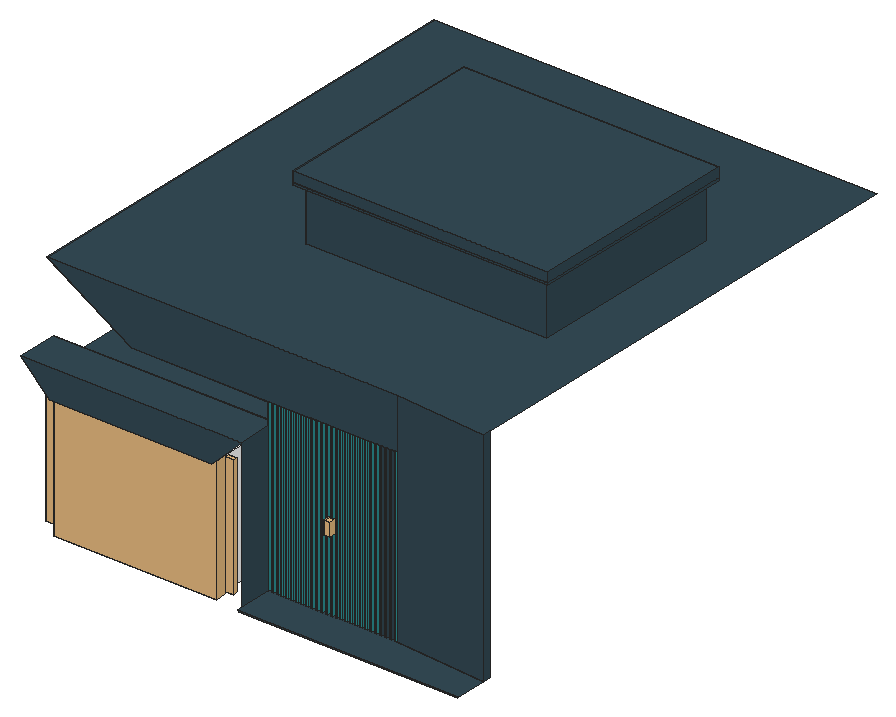
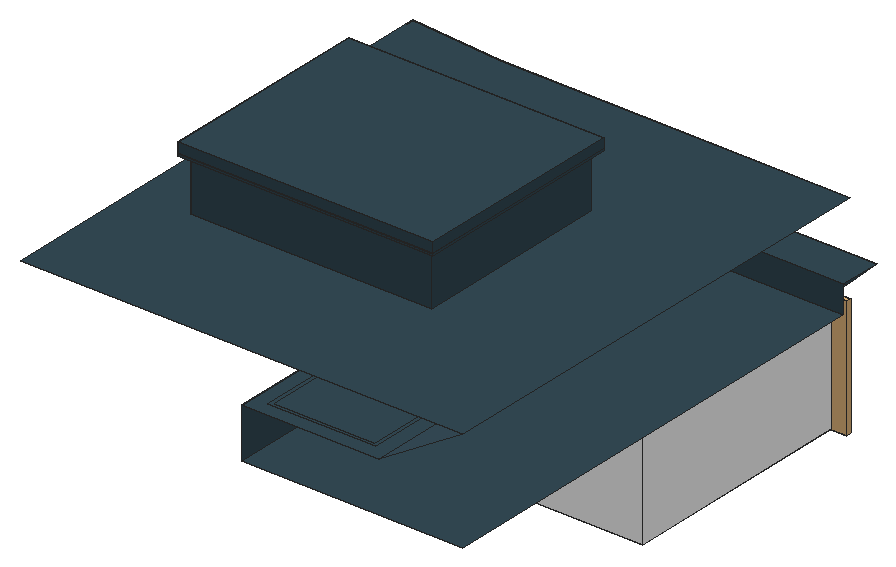
# SketchUp Ruby script. Lengths in inches.
U = 1.inch
M = Sketchup.active_model
def pt(a) = Geom::Point3d.new(a.map { |v| v * U })
def face(e, loops, mat)
  f = e.add_face(loops[0].map { |a| pt(a) })
  loops[1..].each { |l| e.add_face(l.map { |a| pt(a) }).erase! }
  f.material = f.back_material = mat if mat
  f
end
# faces: each face lists its corners as indices into pts; further lists are holes
def faces(e, pts, list, mat = nil) = list.each { |f| face(e, (f[0].is_a?(Array) ? f : [f]).map { |l| l.map { |i| pts[i] } }, mat) }
# xy, xz, yz: faces in a plane at the given z, y or x. An outline is a flat list of corners, or four numbers for a rectangle; further outlines are holes
def ring(l) = l.size == 4 ? [[l[0], l[1]], [l[2], l[1]], [l[2], l[3]], [l[0], l[3]]] : l.each_slice(2).to_a
def flat(e, list, mat, &to3) = list.each { |f| face(e, (f[0].is_a?(Array) ? f : [f]).map { |l| ring(l).map { |u, v| to3.(u, v) } }, mat) }
def xy(e, z, list, mat = nil) = flat(e, list, mat) { |x, y| [x, y, z] }
def xz(e, y, list, mat = nil) = flat(e, list, mat) { |x, z| [x, y, z] }
def yz(e, x, list, mat = nil) = flat(e, list, mat) { |y, z| [x, y, z] }
def lines(e, pts, list) = list.each { |a, b| e.add_line(pt(pts[a]), pt(pts[b])) }
# prism: a flat outline (further loops are holes) pulled along v
def prism(e, loops, v, mat = nil)
  f = face(e, loops, mat); d = Geom::Vector3d.new(v.map { |x| x * U })
  f.pushpull(f.normal.samedirection?(d) ? d.length : -d.length)
end
def box(e, o, s, mat = nil) = prism(e, [[o, [o[0] + s[0], o[1], o[2]], [o[0] + s[0], o[1] + s[1], o[2]], [o[0], o[1] + s[1], o[2]]]], [0, 0, s[2]], mat)
def at(x, y, z, deg = 0) = Geom::Transformation.translation(pt([x, y, z])) * Geom::Transformation.rotation(ORIGIN, Z_AXIS, deg.degrees)
def axes(o, x, y, z) = Geom::Transformation.new([*x, 0, *y, 0, *z, 0, *pt(o).to_a, 1])
def part(name) = M.definitions.add(name)
# library, detail: a bought-in or finely detailed component or shape, given as its bounding box
def library(name, o, s) = part(name).tap { |d| box(d.entities, o, s) }
def detail(e, o, s) = box(e.add_group.entities, o, s)
def put(e, d, t, mat = nil) = e.add_instance(d, t).tap { |i| i.material = mat if mat }
def group(e, t, mat = nil) = e.add_group.tap { |g| g.transformation = t; g.material = mat if mat }.entities
root = M.entities
M.materials.add("0466 AP 9679 Little Andaman-N").color = [89, 168, 184]
M.materials.add("0496 AP 9691 Shadow-N").color = [53, 75, 86]
M.materials.add("0502 AP 7454 DEEP TEAL").color = [46, 147, 149]
M.materials.add("[Color M00]").color = [255, 255, 255]
c1 = library("Sliding windows",[335.6875,-0.89,0.35],[144.14,8.85,122.84])
c2 = library("шторы раздвинутые\#1",[23.6875,-79.1875,2.97],[68.3125,79.67,3.21])
c3 = library("DINING SET",[25.27,8.07,0],[68.7,94.48,53.71])
c4 = library("Wall Light 02",[0,0,0],[3.15,6.76,4.53])
c5 = part("Group\#6")
xy(c5.entities,0,[[1.28,0,0.95,0.04,0.64,0.17,0.375,0.375,0.17,0.64,0.04,0.95,0,1.28,0.04,1.61,0.17,1.92,0.375,2.18,0.64,2.39,0.95,2.51,1.28,2.56,1.61,2.51,1.92,2.39,2.18,2.18,2.39,1.92,2.51,1.61,2.56,1.28,2.51,0.95,2.39,0.64,2.18,0.375,1.92,0.17,1.61,0.04]])
c6 = part("Group\#12")
detail(c6.entities,[2.45,2.45,12.38],[4,4,0.32])
put(c6.entities,c5,at(3.17,3.17,12.51),"[Color M00]")
xy(root,133,[[988.11,217.0625,1120.11,414.75]],"0496 AP 9691 Shadow-N")
xy(root,134,[[1145.11,203.25,1323.11,204.25]],"0496 AP 9691 Shadow-N")
xy(root,135,[[1144.11,203.25,1324.11,203.25,1324.11,234.25,1246.68,234.25,1246.68,236.25,1244.68,236.25,1244.68,234.25,1242.68,234.25,1242.68,236.25,1240.68,236.25,1240.68,234.25,1238.68,234.25,1238.68,236.25,1236.68,236.25,1236.68,234.25,1234.68,234.25,1234.68,236.25,1232.68,236.25,1232.68,234.25,1230.68,234.25,1230.68,236.25,1228.68,236.25,1228.68,234.25,1226.68,234.25,1226.68,236.25,1224.68,236.25,1224.68,234.25,1222.68,234.25,1222.68,236.25,1220.68,236.25,1220.68,234.25,1218.68,234.25,1218.68,236.25,1216.68,236.25,1216.68,234.25,1214.68,234.25,1214.68,236.25,1212.68,236.25,1212.68,234.25,1210.68,234.25,1210.68,236.25,1208.68,236.25,1208.68,234.25,1206.68,234.25,1206.68,236.25,1204.68,236.25,1204.68,234.25,1202.68,234.25,1202.68,236.25,1200.68,236.25,1200.68,234.25,1198.68,234.25,1198.68,236.25,1196.68,236.25,1196.68,234.25,1194.68,234.25,1194.68,236.25,1192.68,236.25,1192.68,234.25,1190.68,234.25,1190.68,236.25,1188.68,236.25,1188.68,234.25,1186.68,234.25,1186.68,236.25,1184.68,236.25,1184.68,234.25,1182.68,234.25,1182.68,236.25,1180.68,236.25,1180.68,234.25,1178.68,234.25,1178.68,236.25,1176.68,236.25,1176.68,234.25,1174.68,234.25,1174.68,236.25,1172.68,236.25,1172.68,234.25,1170.68,234.25,1170.68,236.25,1168.68,236.25,1168.68,234.25,1166.68,234.25,1166.68,236.25,1164.68,236.25,1164.68,234.25,1162.68,234.25,1162.68,236.25,1160.68,236.25,1160.68,234.25,1158.68,234.25,1158.68,236.25,1156.68,236.25,1156.68,234.25,1154.68,234.25,1154.68,236.25,1152.68,236.25,1152.68,234.25,1150.68,234.25,1150.68,236.25,1148.68,236.25,1148.68,234.25,1146.68,234.25,1146.68,236.25,1144.68,236.25,1144.68,234.25,1144.11,234.25]],"0496 AP 9691 Shadow-N")
xy(root,135.01,[[1324.11,228.25,1248.68,234.25,1324.11,234.25]],"0496 AP 9691 Shadow-N")
xy(root,231,[[988.11,207.25,1120.11,220.25]],"0496 AP 9691 Shadow-N")
xy(root,231,[[[988.11,220.25,1120.11,414.75],[1004.21,236.35,1104.01,398.65]],[1006.21,238.35,1102.01,396.65]],"[Color M00]")
xy(root,232.625,[[964.11,240.97,1144.11,627.25]],"0496 AP 9691 Shadow-N")
xy(root,255,[[964.11,207.25,1144.11,240.97]],"0496 AP 9691 Shadow-N")
xy(root,272.98,[[[1032.78,234.25,1144.11,627.25],[1044.78,246.25,1132.11,615.25]],[1144.68,234.25,1146.68,236.25],[1148.68,234.25,1150.68,236.25],[1152.68,234.25,1154.68,236.25],[1156.68,234.25,1158.68,236.25],
  [1160.68,234.25,1162.68,236.25],[1164.68,234.25,1166.68,236.25],[1168.68,234.25,1170.68,236.25],[1172.68,234.25,1174.68,236.25],[1176.68,234.25,1178.68,236.25],
  [1180.68,234.25,1182.68,236.25],[1184.68,234.25,1186.68,236.25],[1188.68,234.25,1190.68,236.25],[1192.68,234.25,1194.68,236.25],[1196.68,234.25,1198.68,236.25],
  [1200.68,234.25,1202.68,236.25],[1204.68,234.25,1206.68,236.25],[1208.68,234.25,1210.68,236.25],[1212.68,234.25,1214.68,236.25],[1216.68,234.25,1218.68,236.25],
  [1220.68,234.25,1222.68,236.25],[1224.68,234.25,1226.68,236.25],[1228.68,234.25,1230.68,236.25],[1232.68,234.25,1234.68,236.25],[1236.68,234.25,1238.68,236.25],
  [1240.68,234.25,1242.68,236.25],[1244.68,234.25,1246.68,236.25],[1046.78,248.25,1130.11,613.25]],"0496 AP 9691 Shadow-N")
xy(root,315,[[1324.11,228.25,1324.11,627.25,964.11,627.25,964.11,234.25,1248.68,234.25]],"0496 AP 9691 Shadow-N")
xz(root,207.25,[[988.11,231,1120.11,231,1144.11,255,964.11,255]],"0496 AP 9691 Shadow-N")
xz(root,234.25,[[1248.68,135,1324.11,135.01],[1248.68,135.01,1324.11,272.98],[1032.78,272.98,1248.68,272.98,1248.68,315,964.11,315]],"0496 AP 9691 Shadow-N")
xz(root,234.25,[[1144.11,135,1144.68,272.98],[1146.68,135,1148.68,272.98],[1150.68,135,1152.68,272.98],[1154.68,135,1156.68,272.98],[1158.68,135,1160.68,272.98],
  [1162.68,135,1164.68,272.98],[1166.68,135,1168.68,272.98],[1170.68,135,1172.68,272.98],[1174.68,135,1176.68,272.98],[1178.68,135,1180.68,272.98],
  [1182.68,135,1184.68,272.98],[1186.68,135,1188.68,272.98],[1190.68,135,1192.68,272.98],[1194.68,135,1196.68,272.98],[1198.68,135,1200.68,272.98],
  [1202.68,135,1204.68,272.98],[1206.68,135,1208.68,272.98],[1210.68,135,1212.68,272.98],[1214.68,135,1216.68,272.98],[1218.68,135,1220.68,272.98],
  [1222.68,135,1224.68,272.98],[1226.68,135,1228.68,272.98],[1230.68,135,1232.68,272.98],[1234.68,135,1236.68,272.98],[1238.68,135,1240.68,272.98],
  [1242.68,135,1244.68,272.98],[1246.68,135,1248.68,272.98]],"0502 AP 7454 DEEP TEAL")
xz(root,236.25,[[1144.68,135,1146.68,272.98],[1148.68,135,1150.68,272.98],[1152.68,135,1154.68,272.98],[1156.68,135,1158.68,272.98],[1160.68,135,1162.68,272.98],
  [1164.68,135,1166.68,272.98],[1168.68,135,1170.68,272.98],[1172.68,135,1174.68,272.98],[1176.68,135,1178.68,272.98],[1180.68,135,1182.68,272.98],
  [1184.68,135,1186.68,272.98],[1188.68,135,1190.68,272.98],[1192.68,135,1194.68,272.98],[1196.68,135,1198.68,272.98],[1200.68,135,1202.68,272.98],
  [1204.68,135,1206.68,272.98],[1208.68,135,1210.68,272.98],[1212.68,135,1214.68,272.98],[1216.68,135,1218.68,272.98],[1220.68,135,1222.68,272.98],
  [1224.68,135,1226.68,272.98],[1228.68,135,1230.68,272.98],[1232.68,135,1234.68,272.98],[1236.68,135,1238.68,272.98],[1240.68,135,1242.68,272.98],
  [1244.68,135,1246.68,272.98]],"0502 AP 7454 DEEP TEAL")
xz(root,240.97,[[964.11,232.625,1144.11,255]],"0496 AP 9691 Shadow-N")
xz(root,414.75,[[988.11,133,1120.11,231]],"[Color M00]")
yz(root,988.11,[[220.25,133,414.75,231]],"[Color M00]")
yz(root,1120.11,[[220.25,133,414.75,231]],"[Color M00]")
yz(root,1144.11,[[207.25,135,234.25,255],[240.97,232.625,240.97,255,234.25,255,234.25,272.98,627.25,272.98,627.25,232.625]],"0496 AP 9691 Shadow-N")
yz(root,1144.68,[[234.25,135,236.25,272.98]],"0502 AP 7454 DEEP TEAL")
yz(root,1146.68,[[234.25,135,236.25,272.98]],"0502 AP 7454 DEEP TEAL")
yz(root,1148.68,[[234.25,135,236.25,272.98]],"0502 AP 7454 DEEP TEAL")
yz(root,1150.68,[[234.25,135,236.25,272.98]],"0502 AP 7454 DEEP TEAL")
yz(root,1152.68,[[234.25,135,236.25,272.98]],"0502 AP 7454 DEEP TEAL")
yz(root,1154.68,[[234.25,135,236.25,272.98]],"0502 AP 7454 DEEP TEAL")
yz(root,1156.68,[[234.25,135,236.25,272.98]],"0502 AP 7454 DEEP TEAL")
yz(root,1158.68,[[234.25,135,236.25,272.98]],"0502 AP 7454 DEEP TEAL")
yz(root,1160.68,[[234.25,135,236.25,272.98]],"0502 AP 7454 DEEP TEAL")
yz(root,1162.68,[[234.25,135,236.25,272.98]],"0502 AP 7454 DEEP TEAL")
yz(root,1164.68,[[234.25,135,236.25,272.98]],"0502 AP 7454 DEEP TEAL")
yz(root,1166.68,[[234.25,135,236.25,272.98]],"0502 AP 7454 DEEP TEAL")
yz(root,1168.68,[[234.25,135,236.25,272.98]],"0502 AP 7454 DEEP TEAL")
yz(root,1170.68,[[234.25,135,236.25,272.98]],"0502 AP 7454 DEEP TEAL")
yz(root,1172.68,[[234.25,135,236.25,272.98]],"0502 AP 7454 DEEP TEAL")
yz(root,1174.68,[[234.25,135,236.25,272.98]],"0502 AP 7454 DEEP TEAL")
yz(root,1176.68,[[234.25,135,236.25,272.98]],"0502 AP 7454 DEEP TEAL")
yz(root,1178.68,[[234.25,135,236.25,272.98]],"0466 AP 9679 Little Andaman-N")
yz(root,1180.68,[[234.25,135,236.25,272.98]],"0502 AP 7454 DEEP TEAL")
yz(root,1182.68,[[234.25,135,236.25,272.98]],"0502 AP 7454 DEEP TEAL")
yz(root,1184.68,[[234.25,135,236.25,272.98]],"0502 AP 7454 DEEP TEAL")
yz(root,1186.68,[[234.25,135,236.25,272.98]],"0502 AP 7454 DEEP TEAL")
yz(root,1188.68,[[234.25,135,236.25,272.98]],"0502 AP 7454 DEEP TEAL")
yz(root,1190.68,[[234.25,135,236.25,272.98]],"0502 AP 7454 DEEP TEAL")
yz(root,1192.68,[[234.25,135,236.25,272.98]],"0502 AP 7454 DEEP TEAL")
yz(root,1194.68,[[234.25,135,236.25,272.98]],"0502 AP 7454 DEEP TEAL")
yz(root,1196.68,[[234.25,135,236.25,272.98]],"0502 AP 7454 DEEP TEAL")
yz(root,1198.68,[[234.25,135,236.25,272.98]],"0502 AP 7454 DEEP TEAL")
yz(root,1200.68,[[234.25,135,236.25,272.98]],"0502 AP 7454 DEEP TEAL")
yz(root,1202.68,[[234.25,135,236.25,272.98]],"0502 AP 7454 DEEP TEAL")
yz(root,1204.68,[[234.25,135,236.25,272.98]],"0502 AP 7454 DEEP TEAL")
yz(root,1206.68,[[234.25,135,236.25,272.98]],"0502 AP 7454 DEEP TEAL")
yz(root,1208.68,[[234.25,135,236.25,272.98]],"0502 AP 7454 DEEP TEAL")
yz(root,1210.68,[[234.25,135,236.25,272.98]],"0502 AP 7454 DEEP TEAL")
yz(root,1212.68,[[234.25,135,236.25,272.98]],"0502 AP 7454 DEEP TEAL")
yz(root,1214.68,[[234.25,135,236.25,272.98]],"0502 AP 7454 DEEP TEAL")
yz(root,1216.68,[[234.25,135,236.25,272.98]],"0502 AP 7454 DEEP TEAL")
yz(root,1218.68,[[234.25,135,236.25,272.98]],"0502 AP 7454 DEEP TEAL")
yz(root,1220.68,[[234.25,135,236.25,272.98]],"0502 AP 7454 DEEP TEAL")
yz(root,1222.68,[[234.25,135,236.25,272.98]],"0502 AP 7454 DEEP TEAL")
yz(root,1224.68,[[234.25,135,236.25,272.98]],"0502 AP 7454 DEEP TEAL")
yz(root,1226.68,[[234.25,135,236.25,272.98]],"0502 AP 7454 DEEP TEAL")
yz(root,1228.68,[[234.25,135,236.25,272.98]],"0502 AP 7454 DEEP TEAL")
yz(root,1230.68,[[234.25,135,236.25,272.98]],"0502 AP 7454 DEEP TEAL")
yz(root,1232.68,[[234.25,135,236.25,272.98]],"0502 AP 7454 DEEP TEAL")
yz(root,1234.68,[[234.25,135,236.25,272.98]],"0502 AP 7454 DEEP TEAL")
yz(root,1236.68,[[234.25,135,236.25,272.98]],"0496 AP 9691 Shadow-N")
yz(root,1238.68,[[234.25,135,236.25,272.98]],"0502 AP 7454 DEEP TEAL")
yz(root,1240.68,[[234.25,135,236.25,272.98]],"0496 AP 9691 Shadow-N")
yz(root,1242.68,[[234.25,135,236.25,272.98]],"0502 AP 7454 DEEP TEAL")
yz(root,1244.68,[[234.25,135,236.25,272.98]],"0496 AP 9691 Shadow-N")
yz(root,1246.68,[[234.25,135,236.25,272.98]],"0502 AP 7454 DEEP TEAL")
yz(root,1324.11,[[228.25,135.01,234.25,315]],"0496 AP 9691 Shadow-N")
p = [[1324.11,228.25,315],[1248.68,234.25,315],[1248.68,234.25,272.98],[1248.68,234.25,135.01],[1324.11,228.25,135.01],[1032.78,234.25,272.98],
  [964.11,234.25,315],[964.11,627.25,315],[1032.78,627.25,272.98]]
faces(root,p,[[0,1,2,3,4],[5,6,7,8]],"0496 AP 9691 Shadow-N")
put(root,c1,axes([680.7,212.47,130.15],[0.91577,0,0],[0,1,0],[0,0,0.81866]))
put(root,c2,axes([922.04,226.9,230.41],[2.23186,0,0],[0,0,1.23016],[0,-1.17,0]))
put(root,c3,at(988.11,289.99,133))
put(root,c4,axes([1193.61,234.25,196.02],[1.47532,0,0],[0,0,1.52],[0,-1.2,0]))
put(root,c6,at(992.24,400.86,218.3),"0496 AP 9691 Shadow-N")
put(root,c6,at(992.24,223.62,218.3),"0496 AP 9691 Shadow-N")
g1 = group(root,at(1049.55,223.62,218.3),"0496 AP 9691 Shadow-N")
detail(g1,[2.45,2.45,12.38],[4,4,0.32])
put(g1,c5,at(3.17,3.17,12.51),"[Color M00]")
put(root,c6,at(1104.05,223.62,218.3),"0496 AP 9691 Shadow-N")
put(root,c6,at(1104.05,312.87,218.3),"0496 AP 9691 Shadow-N")
g2 = group(root,at(992.24,314.56,218.3),"0496 AP 9691 Shadow-N")
detail(g2,[2.45,2.45,12.38],[4,4,0.32])
put(g2,c5,at(3.17,3.17,12.51),"[Color M00]")
put(root,c6,at(1104.05,401,218.3),"0496 AP 9691 Shadow-N")
put(root,c6,at(1049.55,445.25,218.3),"0496 AP 9691 Shadow-N")
put(root,c6,at(1104.05,445.25,218.3),"0496 AP 9691 Shadow-N")
put(root,c6,at(992.24,445.25,218.3),"0496 AP 9691 Shadow-N")
put(root,c6,at(1049.12,401,218.3),"0496 AP 9691 Shadow-N")
g3 = group(root,at(1004.21,236.35,231),"0496 AP 9691 Shadow-N")
xy(g3,0,[[[0,0,99.8,162.3],[2,2,97.8,160.3]]],"[Color M00]")
g4 = group(root,at(1044.78,246.25,272.98),"0496 AP 9691 Shadow-N")
xy(g4,0,[[[0,0,87.34,369],[2,2,85.34,367]]])
g5 = group(root,at(1075.61,344.9375,315),"0496 AP 9691 Shadow-N")
xy(g5,43.0625,[[[0,0,207.59,173.5],[2.76,2.76,204.83,170.74]],[[3.16,3.16,204.43,170.34],[6,6,201.59,167.5]],[6,6,201.59,167.5]],"0496 AP 9691 Shadow-N")
xy(g5,44.79,[[0,0,206.88,0.71],[206.88,0,207.59,173.5],[0,0.71,0.71,172.79],[0,172.79,206.88,173.5]],"0496 AP 9691 Shadow-N")
xy(g5,45.0625,[[0,0,206.88,0.71],[206.88,0,207.59,173.5],[0,0.71,0.71,172.79],[0,172.79,206.88,173.5]],"0496 AP 9691 Shadow-N")
xy(g5,53.0625,[[0,0,207.59,173.5]],"0496 AP 9691 Shadow-N")
xz(g5,0,[[0,43.0625,207.59,44.79],[0,45.0625,207.59,53.0625]],"0496 AP 9691 Shadow-N")
xz(g5,0.71,[[0.71,44.79,206.88,45.0625]],"0496 AP 9691 Shadow-N")
xz(g5,6,[[6,0,201.59,43.0625]],"0496 AP 9691 Shadow-N")
xz(g5,167.5,[[6,0,201.59,43.0625]],"0496 AP 9691 Shadow-N")
xz(g5,172.79,[[0.71,44.79,206.88,45.0625]],"0496 AP 9691 Shadow-N")
xz(g5,173.5,[[0,43.0625,207.59,44.79],[0,45.0625,207.59,53.0625]],"0496 AP 9691 Shadow-N")
yz(g5,0,[[0,43.0625,173.5,44.79],[0,45.0625,173.5,53.0625]],"0496 AP 9691 Shadow-N")
yz(g5,0.71,[[0.71,44.79,172.79,45.0625]],"0496 AP 9691 Shadow-N")
yz(g5,6,[[6,0,167.5,43.0625]],"0496 AP 9691 Shadow-N")
yz(g5,201.59,[[6,0,167.5,43.0625]],"0496 AP 9691 Shadow-N")
yz(g5,206.88,[[0.71,44.79,172.79,45.0625]],"0496 AP 9691 Shadow-N")
yz(g5,207.59,[[0,43.0625,173.5,44.79],[0,45.0625,173.5,53.0625]],"0496 AP 9691 Shadow-N")
g6 = group(g5,at(2.76,2.76,43.0625))
xy(g6,0,[[[0,0,202.07,167.97],[0.4,0.4,201.67,167.57]]],"0496 AP 9691 Shadow-N")
